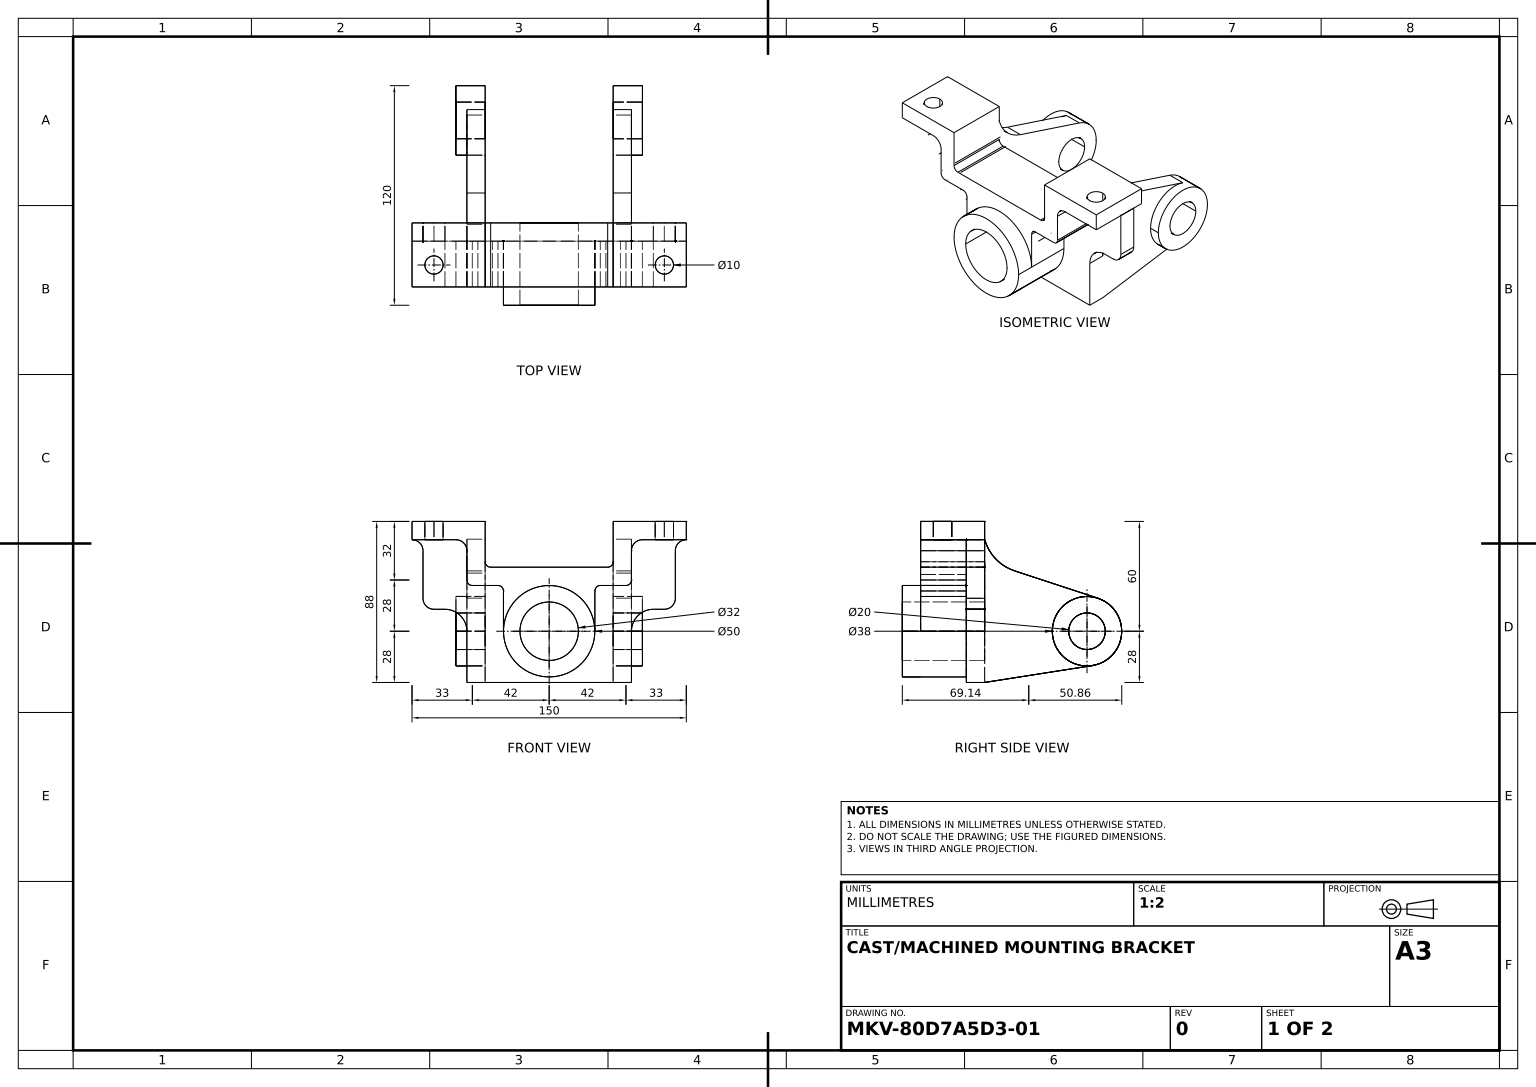
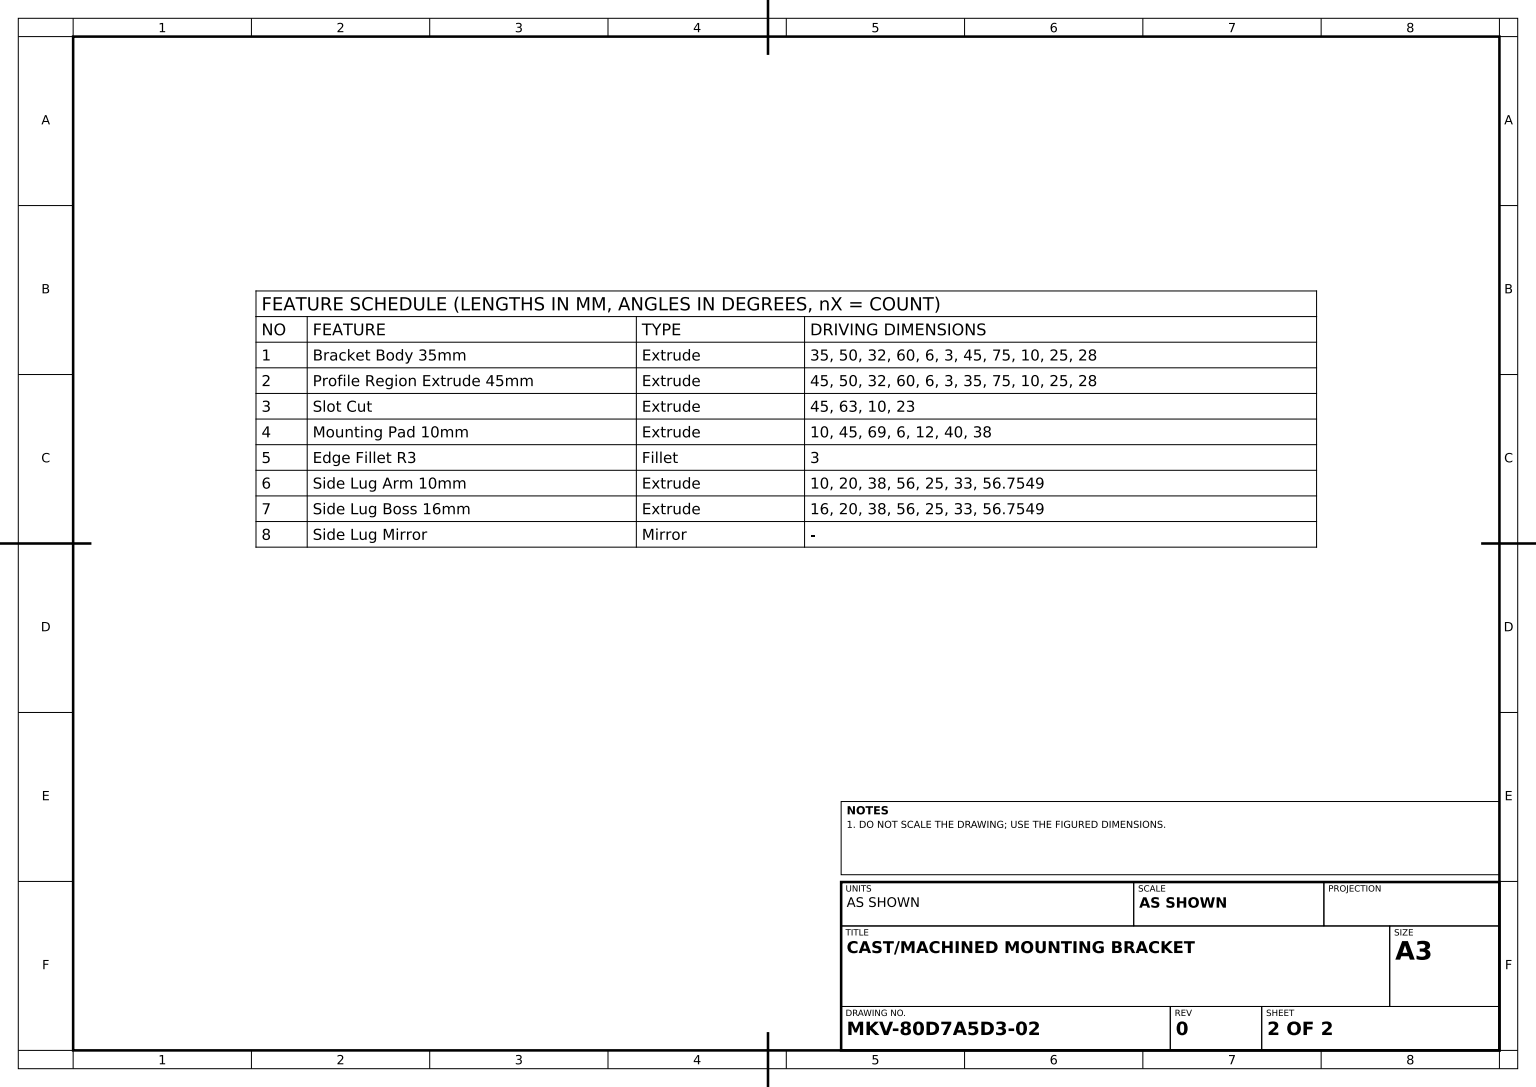
solid
v1 (-45,0,10)
v2 (-45,0,0)
e1 v1 v2 LINE
v3 (-57,12,10)
e2 v1 v3 CIRCLE(AX(P(-57,0,10),D(0,0,1),D(1,0,0)),12)
v4 (-57,12,0)
e3 v3 v4 LINE
e4 v2 v4 CIRCLE(AX(P(-57,0,0),D(0,0,1),D(1,0,0)),12)
face CYL(AX(P(-57,0,10),D(0,0,-1),D(-1,0,0)),12) rev [-e1 e2 e3 -e4]
v5 (75,60,0)
v6 (35,60,0)
e5 v5 v6 LINE
v7 (35,60,35)
e6 v7 v6 LINE
v8 (75,60,35)
e7 v8 v7 LINE
e8 v8 v5 LINE
v9 (63,60,28)
v10 (63,60,18)
e9 v9 v10 CIRCLE(AX(P(63,60,23),D(0,-1,0),D(0,0,-1)),5)
e10 v10 v9 CIRCLE(AX(P(63,60,23),D(0,-1,0),D(0,0,-1)),5)
face PLANE(AX(P(0,60,35),D(0,-1,0),D(0,0,-1))) rev [e5 -e6 -e7 e8] [e9 e10]
v11 (-45,0,-37)
v12 (-45,-18.771282,-58.939212)
e11 v11 v12 CIRCLE(AX(P(-45,0,-56),D(1,0,0),D(0,0,-1)),19)
v13 (-51,0,-37)
e12 v13 v11 LINE
v14 (-51,0,-75)
e13 v13 v14 CIRCLE(AX(P(-51,0,-56),D(1,0,0),D(0,0,-1)),19)
v15 (-35,0,-75)
e14 v14 v15 LINE
v16 (-35,-18.771282,-58.939212)
e15 v16 v15 CIRCLE(AX(P(-35,0,-56),D(1,0,0),D(0,0,-1)),19)
e16 v12 v16 LINE
face CYL(AX(P(-51,0,-56),D(1,0,0),D(0,0,-1)),19) [-e11 -e12 e13 e14 -e15 -e16]
v17 (45,44,10)
v18 (51,50,10)
e17 v17 v18 CIRCLE(AX(P(51,44,10),D(0,0,-1),D(-1,0,0)),6)
v19 (51,50,35)
e18 v19 v18 LINE
v20 (45,44,35)
e19 v20 v19 CIRCLE(AX(P(51,44,35),D(0,0,-1),D(1,0,0)),6)
e20 v20 v17 LINE
face CYL(AX(P(51,44,35),D(0,0,-1),D(-1,0,0)),6) rev [e17 -e18 -e19 e20]
v21 (-45,-28,0)
v22 (-35,-28,0)
e21 v21 v22 LINE
v23 (35,-28,0)
e22 v23 v22 LINE
v24 (45,-28,0)
e23 v24 v23 LINE
v25 (45,-28,10)
e24 v25 v24 LINE
v26 (-45,-28,10)
e25 v25 v26 LINE
e26 v26 v21 LINE
face PLANE(AX(P(-45,-28,10),D(0,-1,0),D(0,0,-1))) [e21 -e22 -e23 -e24 e25 e26]
v27 (45,33,-16.352667)
v28 (45,50.269372,0)
e27 v27 v28 CIRCLE(AX(P(45,56.754858,-24.144119),D(-1,0,0),D(0,0,-1)),25)
v29 (45,0,0)
e28 v29 v28 LINE
v30 (45,0,10)
e29 v30 v29 LINE
e30 v30 v25 LINE
v31 (45,-18.771282,-58.939212)
e31 v31 v24 LINE
v32 (45,0,-37)
e32 v32 v31 CIRCLE(AX(P(45,0,-56),D(1,0,0),D(0,0,-1)),19)
v33 (45,18.053692,-61.921504)
e33 v33 v32 CIRCLE(AX(P(45,0,-56),D(1,0,0),D(0,0,-1)),19)
e34 v33 v27 LINE
face PLANE(AX(P(45,-28,10),D(1,0,0),D(0,0,-1))) [e27 -e28 -e29 e30 e24 -e31 -e32 -e33 e34]
v34 (51,0,-46)
v35 (51,0,-66)
e35 v34 v35 CIRCLE(AX(P(51,0,-56),D(1,0,0),D(0,0,-1)),10)
e36 v35 v34 CIRCLE(AX(P(51,0,-56),D(1,0,0),D(0,0,-1)),10)
v36 (51,0,-75)
v37 (51,0,-37)
e37 v36 v37 CIRCLE(AX(P(51,0,-56),D(1,0,0),D(0,0,-1)),19)
e38 v37 v36 CIRCLE(AX(P(51,0,-56),D(1,0,0),D(0,0,-1)),19)
face PLANE(AX(P(51,0,0),D(-1,0,0),D(0,0,-1))) rev [-e35 -e36] [e37 e38]
v38 (63,50,28)
e39 v9 v38 LINE
v39 (63,50,18)
e40 v38 v39 CIRCLE(AX(P(63,50,23),D(0,-1,0),D(0,0,-1)),5)
e41 v10 v39 LINE
face CYL(AX(P(63,95,23),D(0,-1,0),D(0,0,-1)),5) rev [e39 e40 -e41 -e9]
v40 (25,0,35)
v41 (25,0,10)
e42 v40 v41 LINE
v42 (25,22,10)
e43 v41 v42 LINE
v43 (25,22,35)
e44 v43 v42 LINE
e45 v40 v43 LINE
face PLANE(AX(P(25,0,35),D(-1,0,0),D(0,-1,0))) rev [e42 e43 -e44 -e45]
v44 (42,25,35)
v45 (45,28,35)
e46 v44 v45 CIRCLE(AX(P(42,28,35),D(0,0,1),D(1,0,0)),3)
v46 (42,25,10)
e47 v44 v46 LINE
v47 (45,28,10)
e48 v46 v47 CIRCLE(AX(P(42,28,10),D(0,0,1),D(-1,0,0)),3)
e49 v45 v47 LINE
face CYL(AX(P(42,28,35),D(0,0,-1),D(-1,0,0)),3) [-e46 e47 e48 -e49]
v48 (-25,0,10)
e50 v48 v41 CIRCLE(AX(P(0,0,10),D(0,0,1),D(-1,0,0)),25)
v49 (25,0,45)
e51 v49 v40 LINE
v50 (-25,0,45)
e52 v50 v49 CIRCLE(AX(P(0,0,45),D(0,0,1),D(1,0,0)),25)
v51 (-25,0,35)
e53 v50 v51 LINE
e54 v51 v48 LINE
face CYL(AX(P(0,0,45),D(0,0,-1),D(-1,0,0)),25) [e50 -e42 -e51 -e52 e53 e54]
v52 (-28,25,10)
v53 (-25,22,10)
e55 v52 v53 CIRCLE(AX(P(-28,22,10),D(0,0,-1),D(-1,0,0)),3)
v54 (-25,22,35)
e56 v54 v53 LINE
v55 (-28,25,35)
e57 v54 v55 CIRCLE(AX(P(-28,22,35),D(0,0,1),D(1,0,0)),3)
e58 v55 v52 LINE
face CYL(AX(P(-28,22,35),D(0,0,-1),D(-1,0,0)),3) rev [e55 -e56 e57 e58]
e59 v12 v21 LINE
e60 v26 v1 LINE
v56 (-45,50.269372,0)
e61 v2 v56 LINE
v57 (-45,33,-16.352667)
e62 v57 v56 CIRCLE(AX(P(-45,56.754858,-24.144119),D(-1,0,0),D(0,0,-1)),25)
v58 (-45,18.053692,-61.921504)
e63 v58 v57 LINE
e64 v58 v11 CIRCLE(AX(P(-45,0,-56),D(1,0,0),D(0,0,-1)),19)
face PLANE(AX(P(-45,-28,10),D(-1,0,0),D(0,0,1))) [e59 -e26 e60 e1 e61 -e62 -e63 e64 e11]
v59 (35,0,-66)
e65 v35 v59 LINE
v60 (35,0,-46)
e66 v34 v60 LINE
e67 v59 v60 CIRCLE(AX(P(35,0,-56),D(1,0,0),D(0,0,-1)),10)
face CYL(AX(P(51,0,-56),D(-1,0,0),D(0,0,1)),10) rev [-e65 e36 e66 -e67]
e68 v37 v32 LINE
v61 (35,-18.771282,-58.939212)
e69 v31 v61 LINE
v62 (35,0,-75)
e70 v61 v62 CIRCLE(AX(P(35,0,-56),D(1,0,0),D(0,0,-1)),19)
e71 v36 v62 LINE
face CYL(AX(P(51,0,-56),D(-1,0,0),D(0,0,1)),19) [-e38 e68 e32 e69 e70 -e71]
e72 v49 v50 CIRCLE(AX(P(0,0,45),D(0,0,1),D(1,0,0)),25)
v63 (-16,0,45)
v64 (16,0,45)
e73 v63 v64 CIRCLE(AX(P(0,0,45),D(0,0,1),D(1,0,0)),16)
e74 v64 v63 CIRCLE(AX(P(0,0,45),D(0,0,1),D(1,0,0)),16)
face PLANE(AX(P(0,0,45),D(0,0,1),D(1,0,0))) [e72 e52] [-e73 -e74]
v65 (57,12,0)
e75 v65 v29 CIRCLE(AX(P(57,0,0),D(0,0,1),D(-1,0,0)),12)
v66 (57,12,10)
e76 v66 v65 LINE
e77 v66 v30 CIRCLE(AX(P(57,0,10),D(0,0,1),D(-1,0,0)),12)
face CYL(AX(P(57,0,10),D(0,0,-1),D(-1,0,0)),12) rev [e29 -e75 -e76 e77]
v67 (-35,0,-46)
v68 (-35,0,-66)
e78 v67 v68 CIRCLE(AX(P(-35,0,-56),D(1,0,0),D(0,0,-1)),10)
e79 v68 v67 CIRCLE(AX(P(-35,0,-56),D(1,0,0),D(0,0,-1)),10)
e80 v16 v22 LINE
v69 (-35,18.053692,-61.921504)
e81 v15 v69 CIRCLE(AX(P(-35,0,-56),D(1,0,0),D(0,0,-1)),19)
v70 (-35,33,-16.352667)
e82 v69 v70 LINE
v71 (-35,50.269372,0)
e83 v70 v71 CIRCLE(AX(P(-35,56.754858,-24.144119),D(-1,0,0),D(0,0,-1)),25)
v72 (-35,60,0)
e84 v72 v71 LINE
v73 (-35,60,35)
e85 v73 v72 LINE
v74 (-35,38,35)
e86 v73 v74 LINE
v75 (-35,38,0)
e87 v74 v75 LINE
e88 v22 v75 LINE
face PLANE(AX(P(-35,0,35),D(1,0,0),D(0,0,-1))) [-e78 -e79] [-e80 e15 e81 e82 e83 -e84 -e85 e86 e87 -e88]
v76 (-51,0,-66)
v77 (-51,0,-46)
e89 v76 v77 CIRCLE(AX(P(-51,0,-56),D(1,0,0),D(0,0,-1)),10)
e90 v76 v68 LINE
e91 v77 v67 LINE
face CYL(AX(P(-51,0,-56),D(1,0,0),D(0,0,-1)),10) rev [-e89 e90 e79 -e91]
face PLANE(AX(P(-45,-27.329941,-4.27933),D(0,0.987962214,0.154695393),D(0,-0.154695393,0.987962214))) rev [e80 -e21 -e59 e16]
e92 v57 v70 LINE
e93 v58 v69 LINE
face PLANE(AX(P(-45,34.637294,-11.360827),D(0,0.950194313,-0.311658093),D(0,0.311658093,0.950194313))) [e92 -e82 -e93 e63]
v78 (-45,28,35)
v79 (-45,28,10)
e94 v78 v79 LINE
v80 (-45,44,35)
e95 v78 v80 LINE
v81 (-45,44,10)
e96 v80 v81 LINE
e97 v81 v79 LINE
face PLANE(AX(P(-45,0,35),D(-1,0,0),D(0,0,1))) [-e94 e95 e96 e97]
e98 v14 v13 CIRCLE(AX(P(-51,0,-56),D(1,0,0),D(0,0,-1)),19)
e99 v77 v76 CIRCLE(AX(P(-51,0,-56),D(1,0,0),D(0,0,-1)),10)
face PLANE(AX(P(-51,0,0),D(1,0,0),D(0,0,-1))) rev [-e98 -e13] [e89 e99]
v82 (63,12,10)
e100 v82 v66 LINE
v83 (63,12,0)
e101 v83 v65 LINE
e102 v82 v83 LINE
face PLANE(AX(P(57,12,10),D(0,-1,0),D(0,0,-1))) [e100 e76 -e101 -e102]
v84 (-63,50,28)
v85 (-63,50,18)
e103 v84 v85 CIRCLE(AX(P(-63,50,23),D(0,-1,0),D(0,0,1)),5)
e104 v85 v84 CIRCLE(AX(P(-63,50,23),D(0,-1,0),D(0,0,1)),5)
v86 (-75,50,35)
v87 (-75,50,10)
e105 v86 v87 LINE
v88 (-51,50,10)
e106 v87 v88 LINE
v89 (-51,50,35)
e107 v89 v88 LINE
e108 v89 v86 LINE
face PLANE(AX(P(0,50,35),D(0,-1,0),D(0,0,-1))) [-e103 -e104] [e105 e106 -e107 e108]
v90 (75,50,10)
v91 (75,50,0)
e109 v90 v91 LINE
e110 v91 v5 LINE
v92 (75,50,35)
e111 v92 v8 LINE
e112 v92 v90 LINE
face PLANE(AX(P(75,0,35),D(-1,0,0),D(0,0,1))) rev [e109 e110 -e8 -e111 e112]
v93 (-75,50,0)
v94 (-75,60,0)
e113 v93 v94 LINE
e114 v87 v93 LINE
v95 (-75,60,35)
e115 v86 v95 LINE
e116 v95 v94 LINE
face PLANE(AX(P(-75,0,35),D(-1,0,0),D(0,0,1))) [-e113 -e114 -e105 e115 e116]
v96 (-63,12,0)
e117 v4 v96 LINE
v97 (-69,18,0)
e118 v96 v97 CIRCLE(AX(P(-63,18,0),D(0,0,-1),D(-1,0,0)),6)
v98 (-69,44,0)
e119 v97 v98 LINE
e120 v98 v93 CIRCLE(AX(P(-75,44,0),D(0,0,1),D(-1,0,0)),6)
e121 v94 v72 LINE
e122 v56 v71 LINE
face PLANE(AX(P(0,0,0),D(0,0,1),D(1,0,0))) rev [e117 e118 e119 e120 e113 e121 e84 -e122 -e61 e4]
v99 (-32,35,35)
v100 (32,35,35)
e123 v99 v100 LINE
e124 v99 v74 CIRCLE(AX(P(-32,38,35),D(0,0,-1),D(1,0,0)),3)
e125 v95 v73 LINE
e126 v80 v89 CIRCLE(AX(P(-51,44,35),D(0,0,1),D(1,0,0)),6)
v101 (-42,25,35)
e127 v101 v78 CIRCLE(AX(P(-42,28,35),D(0,0,-1),D(1,0,0)),3)
e128 v55 v101 LINE
e129 v51 v54 LINE
e130 v40 v51 CIRCLE(AX(P(0,0,35),D(0,0,1),D(1,0,0)),25)
v102 (28,25,35)
e131 v43 v102 CIRCLE(AX(P(28,22,35),D(0,0,-1),D(1,0,0)),3)
e132 v102 v44 LINE
e133 v45 v20 LINE
e134 v19 v92 LINE
v103 (35,38,35)
e135 v7 v103 LINE
e136 v103 v100 CIRCLE(AX(P(32,38,35),D(0,0,-1),D(1,0,0)),3)
face PLANE(AX(P(0,0,35),D(0,0,1),D(1,0,0))) [-e123 e124 -e86 -e125 -e115 -e108 -e126 -e95 -e127 -e128 -e57 -e129 -e130 e45 e131 e132 e46 e133 e19 e134 e111 e7 e135 e136]
v104 (-42,25,10)
e137 v79 v104 CIRCLE(AX(P(-42,28,10),D(0,0,1),D(-1,0,0)),3)
e138 v101 v104 LINE
face CYL(AX(P(-42,28,35),D(0,0,-1),D(-1,0,0)),3) [e137 -e138 e127 e94]
v105 (-63,12,10)
e139 v3 v105 LINE
e140 v105 v96 LINE
face PLANE(AX(P(-57,12,10),D(0,-1,0),D(0,0,-1))) [-e117 -e3 e139 e140]
v106 (69,44,10)
v107 (69,44,0)
e141 v106 v107 LINE
v108 (69,18,10)
e142 v106 v108 LINE
v109 (69,18,0)
e143 v108 v109 LINE
e144 v107 v109 LINE
face PLANE(AX(P(69,18,10),D(1,0,0),D(0,0,-1))) [-e141 e142 e143 -e144]
v110 (35,33,-16.352667)
e145 v27 v110 LINE
v111 (35,18.053692,-61.921504)
e146 v33 v111 LINE
e147 v111 v110 LINE
face PLANE(AX(P(45,34.637294,-11.360827),D(0,-0.950194313,0.311658093),D(0,-0.311658093,-0.950194313))) rev [-e145 -e34 e146 e147]
e148 v47 v17 LINE
face PLANE(AX(P(45,0,35),D(-1,0,0),D(0,0,1))) rev [e49 e148 -e20 -e133]
e149 v53 v48 LINE
face PLANE(AX(P(-25,0,35),D(-1,0,0),D(0,-1,0))) [e129 e56 e149 -e54]
v112 (-63,60,28)
v113 (-63,60,18)
e150 v112 v113 CIRCLE(AX(P(-63,60,23),D(0,1,0),D(0,0,1)),5)
e151 v113 v112 CIRCLE(AX(P(-63,60,23),D(0,1,0),D(0,0,1)),5)
face PLANE(AX(P(0,60,35),D(0,1,0),D(0,0,1))) [e125 e85 -e121 -e116] [-e150 -e151]
face CYL(AX(P(-51,0,-56),D(1,0,0),D(0,0,-1)),10) rev [-e99 e91 e78 -e90]
v114 (35,50.269372,0)
e152 v28 v114 LINE
e153 v6 v114 LINE
e154 v91 v107 CIRCLE(AX(P(75,44,0),D(0,0,1),D(1,0,0)),6)
e155 v109 v83 CIRCLE(AX(P(63,18,0),D(0,0,-1),D(1,0,0)),6)
face PLANE(AX(P(0,0,0),D(0,0,1),D(1,0,0))) rev [e101 e75 e28 e152 -e153 -e5 -e110 e154 e144 e155]
v115 (-69,18,10)
e156 v105 v115 CIRCLE(AX(P(-63,18,10),D(0,0,-1),D(-1,0,0)),6)
e157 v115 v97 LINE
face CYL(AX(P(-63,18,10),D(0,0,-1),D(-1,0,0)),6) [-e140 e156 e157 -e118]
v116 (-32,35,0)
e158 v116 v99 LINE
e159 v75 v116 CIRCLE(AX(P(-32,38,0),D(0,0,1),D(1,0,0)),3)
face CYL(AX(P(-32,38,35),D(0,0,1),D(1,0,0)),3) rev [-e158 -e159 -e87 -e124]
e160 v112 v84 LINE
e161 v113 v85 LINE
face CYL(AX(P(-63,95,23),D(0,-1,0),D(0,0,-1)),5) rev [-e160 e150 e161 e104]
face CYL(AX(P(-51,0,-56),D(1,0,0),D(0,0,-1)),19) [-e81 -e14 e98 e12 -e64 e93]
v117 (-69,44,10)
e162 v117 v98 LINE
e163 v115 v117 LINE
face PLANE(AX(P(-69,18,10),D(-1,0,0),D(0,0,1))) [e162 -e119 -e157 e163]
e164 v104 v52 LINE
face PLANE(AX(P(0,25,35),D(0,-1,0),D(1,0,0))) [e164 -e58 e128 e138]
v118 (28,25,10)
e165 v42 v118 CIRCLE(AX(P(28,22,10),D(0,0,-1),D(-1,0,0)),3)
e166 v102 v118 LINE
face CYL(AX(P(28,22,35),D(0,0,-1),D(-1,0,0)),3) rev [-e131 e44 e165 -e166]
e167 v90 v106 CIRCLE(AX(P(75,44,10),D(0,0,1),D(1,0,0)),6)
face CYL(AX(P(75,44,10),D(0,0,-1),D(-1,0,0)),6) rev [e167 e141 -e154 -e109]
e168 v88 v81 CIRCLE(AX(P(-51,44,10),D(0,0,-1),D(-1,0,0)),6)
face CYL(AX(P(-51,44,35),D(0,0,-1),D(-1,0,0)),6) rev [e107 e168 -e96 e126]
e169 v39 v38 CIRCLE(AX(P(63,50,23),D(0,-1,0),D(0,0,-1)),5)
e170 v18 v90 LINE
face PLANE(AX(P(0,50,35),D(0,1,0),D(0,0,1))) rev [-e169 -e40] [-e112 -e134 e18 e170]
e171 v117 v87 CIRCLE(AX(P(-75,44,10),D(0,0,1),D(-1,0,0)),6)
face CYL(AX(P(-75,44,10),D(0,0,-1),D(-1,0,0)),6) rev [e171 e114 -e120 -e162]
e172 v110 v114 CIRCLE(AX(P(35,56.754858,-24.144119),D(-1,0,0),D(0,0,-1)),25)
face CYL(AX(P(45,56.754858,-24.144119),D(-1,0,0),D(0,0,1)),25) rev [-e152 -e27 e145 e172]
e173 v108 v82 CIRCLE(AX(P(63,18,10),D(0,0,-1),D(1,0,0)),6)
e174 v118 v46 LINE
face PLANE(AX(P(-51,44,10),D(0,0,-1),D(-1,0,0))) rev [-e164 -e137 -e97 -e168 -e106 -e171 -e163 -e156 -e139 -e2 -e60 -e25 -e30 -e77 -e100 -e173 -e142 -e167 -e170 -e17 -e148 -e48 -e174 -e165 -e43 -e50 -e149 -e55]
face CYL(AX(P(-45,56.754858,-24.144119),D(1,0,0),D(0,0,-1)),25) rev [e62 e122 -e83 -e92]
e175 v62 v111 CIRCLE(AX(P(35,0,-56),D(1,0,0),D(0,0,-1)),19)
face CYL(AX(P(51,0,-56),D(-1,0,0),D(0,0,1)),19) [e33 -e68 -e37 e71 e175 -e146]
face CYL(AX(P(63,95,23),D(0,-1,0),D(0,0,-1)),5) rev [e169 -e39 -e10 e41]
v119 (16,0,0)
e176 v64 v119 LINE
v120 (-16,0,0)
e177 v120 v119 CIRCLE(AX(P(0,0,0),D(0,0,1),D(1,0,0)),16)
e178 v63 v120 LINE
face CYL(AX(P(0,0,45),D(0,0,-1),D(-1,0,0)),16) rev [e73 e176 -e177 -e178]
face CYL(AX(P(-63,95,23),D(0,-1,0),D(0,0,-1)),5) rev [-e161 e151 e160 e103]
e179 v61 v23 LINE
face PLANE(AX(P(45,-27.329941,-4.27933),D(0,-0.987962214,-0.154695393),D(0,0.154695393,-0.987962214))) [e31 e23 -e179 -e69]
v121 (32,35,0)
e180 v116 v121 LINE
v122 (35,38,0)
e181 v121 v122 CIRCLE(AX(P(32,38,0),D(0,0,1),D(1,0,0)),3)
e182 v23 v122 LINE
e183 v119 v120 CIRCLE(AX(P(0,0,0),D(0,0,1),D(1,0,0)),16)
face PLANE(AX(P(0,0,0),D(0,0,1),D(1,0,0))) rev [e180 e181 -e182 e22 e88 e159] [e183 e177]
e184 v60 v59 CIRCLE(AX(P(35,0,-56),D(1,0,0),D(0,0,-1)),10)
face CYL(AX(P(51,0,-56),D(-1,0,0),D(0,0,1)),10) rev [-e184 -e66 e35 e65]
face PLANE(AX(P(0,25,35),D(0,1,0),D(-1,0,0))) rev [-e132 e166 e174 -e47]
e185 v122 v103 LINE
face PLANE(AX(P(35,0,35),D(1,0,0),D(0,0,-1))) rev [e6 e153 -e172 -e147 -e175 -e70 e179 e182 e185 -e135] [e67 e184]
face CYL(AX(P(0,0,45),D(0,0,-1),D(-1,0,0)),25) [-e53 -e72 e51 e130]
e186 v100 v121 LINE
face CYL(AX(P(32,38,35),D(0,0,-1),D(-1,0,0)),3) rev [-e136 -e185 -e181 -e186]
face CYL(AX(P(0,0,45),D(0,0,-1),D(-1,0,0)),16) rev [e74 e178 -e183 -e176]
face PLANE(AX(P(0,35,35),D(0,1,0),D(0,0,1))) [e158 e123 e186 -e180]
face CYL(AX(P(63,18,10),D(0,0,-1),D(-1,0,0)),6) [e102 -e155 -e143 e173]
